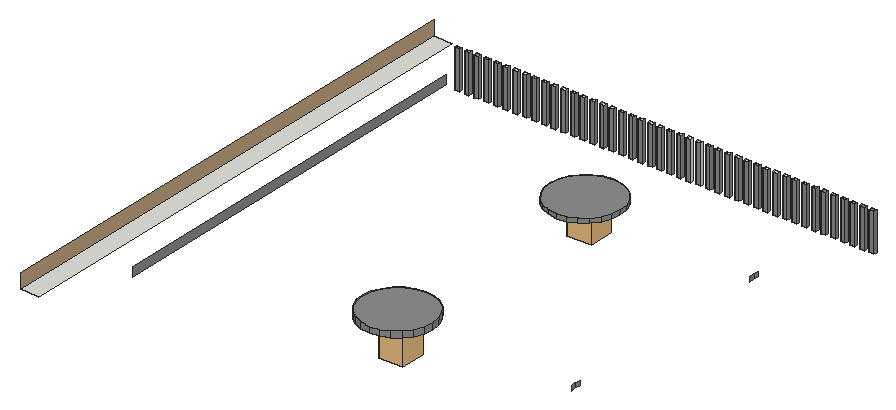
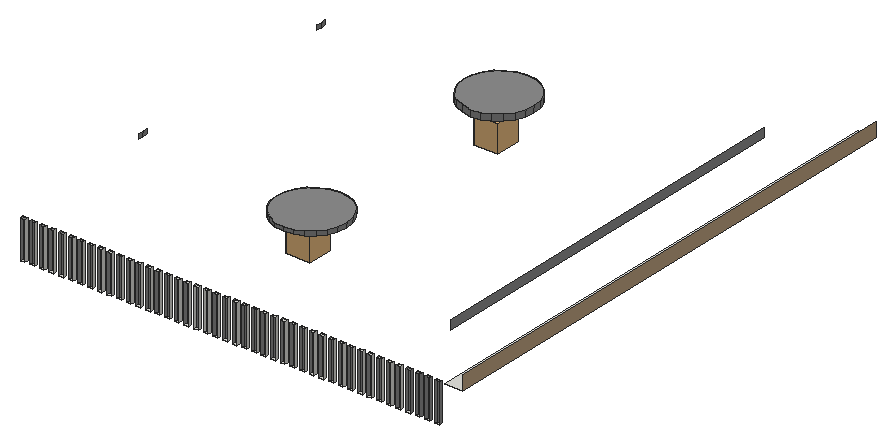
# SketchUp Ruby script. Lengths in inches.
U = 1.inch
M = Sketchup.active_model
def pt(a) = Geom::Point3d.new(a.map { |v| v * U })
def face(e, loops, mat)
  f = e.add_face(loops[0].map { |a| pt(a) })
  loops[1..].each { |l| e.add_face(l.map { |a| pt(a) }).erase! }
  f.material = f.back_material = mat if mat
  f
end
# faces: each face lists its corners as indices into pts; further lists are holes
def faces(e, pts, list, mat = nil) = list.each { |f| face(e, (f[0].is_a?(Array) ? f : [f]).map { |l| l.map { |i| pts[i] } }, mat) }
# xy, xz, yz: faces in a plane at the given z, y or x. An outline is a flat list of corners, or four numbers for a rectangle; further outlines are holes
def ring(l) = l.size == 4 ? [[l[0], l[1]], [l[2], l[1]], [l[2], l[3]], [l[0], l[3]]] : l.each_slice(2).to_a
def flat(e, list, mat, &to3) = list.each { |f| face(e, (f[0].is_a?(Array) ? f : [f]).map { |l| ring(l).map { |u, v| to3.(u, v) } }, mat) }
def xy(e, z, list, mat = nil) = flat(e, list, mat) { |x, y| [x, y, z] }
def xz(e, y, list, mat = nil) = flat(e, list, mat) { |x, z| [x, y, z] }
def yz(e, x, list, mat = nil) = flat(e, list, mat) { |y, z| [x, y, z] }
def lines(e, pts, list) = list.each { |a, b| e.add_line(pt(pts[a]), pt(pts[b])) }
# prism: a flat outline (further loops are holes) pulled along v
def prism(e, loops, v, mat = nil)
  f = face(e, loops, mat); d = Geom::Vector3d.new(v.map { |x| x * U })
  f.pushpull(f.normal.samedirection?(d) ? d.length : -d.length)
end
def box(e, o, s, mat = nil) = prism(e, [[o, [o[0] + s[0], o[1], o[2]], [o[0] + s[0], o[1] + s[1], o[2]], [o[0], o[1] + s[1], o[2]]]], [0, 0, s[2]], mat)
def at(x, y, z, deg = 0) = Geom::Transformation.translation(pt([x, y, z])) * Geom::Transformation.rotation(ORIGIN, Z_AXIS, deg.degrees)
def axes(o, x, y, z) = Geom::Transformation.new([*x, 0, *y, 0, *z, 0, *pt(o).to_a, 1])
def part(name) = M.definitions.add(name)
# library, detail: a bought-in or finely detailed component or shape, given as its bounding box
def library(name, o, s) = part(name).tap { |d| box(d.entities, o, s) }
def detail(e, o, s) = box(e.add_group.entities, o, s)
def put(e, d, t, mat = nil) = e.add_instance(d, t).tap { |i| i.material = mat if mat }
def group(e, t, mat = nil) = e.add_group.tap { |g| g.transformation = t; g.material = mat if mat }.entities
root = M.entities
M.materials.add("Sand A01 200cm").color = [193, 166, 131]
M.materials.add("[Color M04]").color = [142, 142, 142]
c1 = library("Spot Light\#4",[-5.1,-5.1,-11.05],[10.2,10.2,11.05])
c2 = library("Spot Light\#3",[-5.1,-5.1,-11.05],[10.2,10.2,11.05])
xy(root,222.8125,[[20.94,222.56,22.88,223.75],[24.91,222.56,26.85,223.75],[28.88,222.56,30.82,223.75],[32.85,222.56,34.79,223.75],[36.82,222.56,38.76,223.75],
  [40.79,222.56,42.73,223.75],[44.76,222.56,46.7,223.75],[48.73,222.56,50.67,223.75],[52.7,222.56,54.64,223.75],[56.67,222.56,58.61,223.75],
  [60.64,222.56,62.58,223.75],[64.6,222.56,66.55,223.75],[68.57,222.56,70.52,223.75],[72.54,222.56,74.49,223.75],[76.51,222.56,78.45,223.75],
  [80.48,222.56,82.42,223.75],[84.45,222.56,86.39,223.75],[88.42,222.56,90.36,223.75],[92.39,222.56,94.33,223.75],[96.36,222.56,98.3,223.75],
  [100.33,222.56,102.27,223.75],[104.3,222.56,106.24,223.75],[108.27,222.56,110.21,223.75],[112.24,222.56,114.18,223.75],[116.21,222.56,118.15,223.75],
  [120.18,222.56,122.12,223.75],[124.14,222.56,126.09,223.75],[128.11,222.56,130.06,223.75],[132.08,222.56,134.03,223.75],[136.05,222.56,137.99,223.75],
  [140.02,222.56,141.96,223.75],[143.99,222.56,145.93,223.75],[147.96,222.56,149.9,223.75],[151.93,222.56,153.87,223.75],[155.9,222.56,157.84,223.75],
  [159.87,222.56,161.81,223.75],[163.84,222.56,165.78,223.75],[167.81,222.56,169.75,223.75],[171.78,222.56,173.72,223.75],[175.75,222.56,177.6875,223.75],
  [179.71,222.56,181.66,223.75],[183.68,222.56,185.625,223.75],[187.65,222.56,189.6,223.75],[191.62,222.56,193.56,223.75]])
xy(root,238.625,[[11.13,11.13,18.94,223.75],[36.82,222.56,38.76,223.75],[40.79,222.56,42.73,223.75],[44.76,222.56,46.7,223.75],[48.73,222.56,50.67,223.75],
  [52.7,222.56,54.64,223.75],[56.67,222.56,58.61,223.75],[60.64,222.56,62.58,223.75],[64.6,222.56,66.55,223.75],[68.57,222.56,70.52,223.75],
  [72.54,222.56,74.49,223.75],[76.51,222.56,78.45,223.75],[80.48,222.56,82.42,223.75],[84.45,222.56,86.39,223.75],[88.42,222.56,90.36,223.75],
  [92.39,222.56,94.33,223.75],[96.36,222.56,98.3,223.75],[100.33,222.56,102.27,223.75],[104.3,222.56,106.24,223.75],[108.27,222.56,110.21,223.75],
  [112.24,222.56,114.18,223.75],[116.21,222.56,118.15,223.75],[120.18,222.56,122.12,223.75],[124.14,222.56,126.09,223.75],[128.11,222.56,130.06,223.75],
  [132.08,222.56,134.03,223.75],[136.05,222.56,137.99,223.75],[140.02,222.56,141.96,223.75],[143.99,222.56,145.93,223.75],[147.96,222.56,149.9,223.75],
  [151.93,222.56,153.87,223.75],[155.9,222.56,157.84,223.75],[159.87,222.56,161.81,223.75],[163.84,222.56,165.78,223.75]])
xy(root,238.625,[[20.94,222.56,22.88,223.75],[24.91,222.56,26.85,223.75],[28.88,222.56,30.82,223.75],[32.85,222.56,34.79,223.75],[167.81,222.56,169.75,223.75],
  [171.78,222.56,173.72,223.75],[175.75,222.56,177.6875,223.75],[179.71,222.56,181.66,223.75],[183.68,222.56,185.625,223.75],[187.65,222.56,189.6,223.75],
  [191.62,222.56,193.56,223.75]],"[Color M04]")
xy(root,242.625,[[119.36,152.06,115.61,152.55,112.11,154,109.11,156.31,106.8,159.31,105.35,162.81,104.86,166.56,105.35,170.3125,106.8,173.81,109.11,176.8125,112.11,179.12,115.61,180.57,119.36,181.06,123.11,180.57,126.61,179.12,129.61,176.8125,131.92,173.81,133.37,170.3125,133.86,166.56,133.37,162.81,131.92,159.31,129.61,156.31,126.61,154,123.11,152.55]],"[Color M04]")
xy(root,243.4375,[[119.36,55.56,115.61,56.05,112.11,57.5,109.11,59.81,106.8,62.81,105.35,66.31,104.86,70.06,105.35,73.8125,106.8,77.31,109.11,80.3125,112.11,82.62,115.61,84.07,119.36,84.56,123.11,84.07,126.61,82.62,129.61,80.3125,131.92,77.31,133.37,73.8125,133.86,70.06,133.37,66.31,131.92,62.81,129.61,59.81,126.61,57.5,123.11,56.05]],"[Color M04]")
xz(root,222.56,[[20.94,222.8125,22.88,238.625],[24.91,222.8125,26.85,238.625],[28.88,222.8125,30.82,238.625],[32.85,222.8125,34.79,238.625],[36.82,222.8125,38.76,238.625],
  [40.79,222.8125,42.73,238.625],[44.76,222.8125,46.7,238.625],[48.73,222.8125,50.67,238.625],[52.7,222.8125,54.64,238.625],[56.67,222.8125,58.61,238.625],
  [60.64,222.8125,62.58,238.625],[64.6,222.8125,66.55,238.625],[68.57,222.8125,70.52,238.625],[72.54,222.8125,74.49,238.625],[76.51,222.8125,78.45,238.625],
  [80.48,222.8125,82.42,238.625],[84.45,222.8125,86.39,238.625],[88.42,222.8125,90.36,238.625],[92.39,222.8125,94.33,238.625],[96.36,222.8125,98.3,238.625],
  [100.33,222.8125,102.27,238.625],[104.3,222.8125,106.24,238.625],[108.27,222.8125,110.21,238.625],[112.24,222.8125,114.18,238.625],[116.21,222.8125,118.15,238.625],
  [120.18,222.8125,122.12,238.625],[124.14,222.8125,126.09,238.625],[128.11,222.8125,130.06,238.625],[132.08,222.8125,134.03,238.625],[136.05,222.8125,137.99,238.625],
  [140.02,222.8125,141.96,238.625],[143.99,222.8125,145.93,238.625],[147.96,222.8125,149.9,238.625],[151.93,222.8125,153.87,238.625],[155.9,222.8125,157.84,238.625],
  [159.87,222.8125,161.81,238.625],[163.84,222.8125,165.78,238.625],[167.81,222.8125,169.75,238.625],[171.78,222.8125,173.72,238.625],[175.75,222.8125,177.6875,238.625],
  [179.71,222.8125,181.66,238.625],[183.68,222.8125,185.625,238.625],[187.65,222.8125,189.6,238.625],[191.62,222.8125,193.56,238.625]],"[Color M04]")
yz(root,11.13,[[11.13,238.625,223.75,244.625]],"Sand A01 200cm")
yz(root,20.94,[[222.56,222.8125,223.75,238.625]],"[Color M04]")
yz(root,22.88,[[222.56,222.8125,223.75,238.625]],"[Color M04]")
yz(root,24.91,[[222.56,222.8125,223.75,238.625]],"[Color M04]")
yz(root,26.85,[[222.56,222.8125,223.75,238.625]],"[Color M04]")
yz(root,28.88,[[222.56,222.8125,223.75,238.625]],"[Color M04]")
yz(root,30.82,[[222.56,222.8125,223.75,238.625]],"[Color M04]")
yz(root,32.85,[[222.56,222.8125,223.75,238.625]],"[Color M04]")
yz(root,34.79,[[222.56,222.8125,223.75,238.625]],"[Color M04]")
yz(root,36.82,[[222.56,222.8125,223.75,238.625]])
yz(root,36.86,[[36.86,240.875,198.01,244.625]],"[Color M04]")
yz(root,38.76,[[222.56,222.8125,223.75,238.625]],"[Color M04]")
yz(root,40.79,[[222.56,222.8125,223.75,238.625]])
yz(root,42.73,[[222.56,222.8125,223.75,238.625]],"[Color M04]")
yz(root,44.76,[[222.56,222.8125,223.75,238.625]])
yz(root,46.7,[[222.56,222.8125,223.75,238.625]],"[Color M04]")
yz(root,48.73,[[222.56,222.8125,223.75,238.625]])
yz(root,50.67,[[222.56,222.8125,223.75,238.625]],"[Color M04]")
yz(root,52.7,[[222.56,222.8125,223.75,238.625]])
yz(root,54.64,[[222.56,222.8125,223.75,238.625]],"[Color M04]")
yz(root,56.67,[[222.56,222.8125,223.75,238.625]])
yz(root,58.61,[[222.56,222.8125,223.75,238.625]],"[Color M04]")
yz(root,60.64,[[222.56,222.8125,223.75,238.625]])
yz(root,62.58,[[222.56,222.8125,223.75,238.625]],"[Color M04]")
yz(root,64.6,[[222.56,222.8125,223.75,238.625]])
yz(root,66.55,[[222.56,222.8125,223.75,238.625]],"[Color M04]")
yz(root,68.57,[[222.56,222.8125,223.75,238.625]])
yz(root,70.52,[[222.56,222.8125,223.75,238.625]],"[Color M04]")
yz(root,72.54,[[222.56,222.8125,223.75,238.625]])
yz(root,74.49,[[222.56,222.8125,223.75,238.625]],"[Color M04]")
yz(root,76.51,[[222.56,222.8125,223.75,238.625]])
yz(root,78.45,[[222.56,222.8125,223.75,238.625]],"[Color M04]")
yz(root,80.48,[[222.56,222.8125,223.75,238.625]])
yz(root,82.42,[[222.56,222.8125,223.75,238.625]],"[Color M04]")
yz(root,84.45,[[222.56,222.8125,223.75,238.625]])
yz(root,86.39,[[222.56,222.8125,223.75,238.625]],"[Color M04]")
yz(root,88.42,[[222.56,222.8125,223.75,238.625]])
yz(root,90.36,[[222.56,222.8125,223.75,238.625]],"[Color M04]")
yz(root,92.39,[[222.56,222.8125,223.75,238.625]])
yz(root,94.33,[[222.56,222.8125,223.75,238.625]],"[Color M04]")
yz(root,96.36,[[222.56,222.8125,223.75,238.625]])
yz(root,98.3,[[222.56,222.8125,223.75,238.625]],"[Color M04]")
yz(root,100.33,[[222.56,222.8125,223.75,238.625]])
yz(root,102.27,[[222.56,222.8125,223.75,238.625]],"[Color M04]")
yz(root,104.3,[[222.56,222.8125,223.75,238.625]])
yz(root,106.24,[[222.56,222.8125,223.75,238.625]],"[Color M04]")
yz(root,108.27,[[222.56,222.8125,223.75,238.625]])
yz(root,110.21,[[222.56,222.8125,223.75,238.625]],"[Color M04]")
yz(root,112.24,[[222.56,222.8125,223.75,238.625]])
yz(root,114.18,[[222.56,222.8125,223.75,238.625]],"[Color M04]")
yz(root,116.21,[[222.56,222.8125,223.75,238.625]])
yz(root,118.15,[[222.56,222.8125,223.75,238.625]])
yz(root,120.18,[[222.56,222.8125,223.75,238.625]])
yz(root,122.12,[[222.56,222.8125,223.75,238.625]])
yz(root,124.14,[[222.56,222.8125,223.75,238.625]])
yz(root,126.09,[[222.56,222.8125,223.75,238.625]],"[Color M04]")
yz(root,128.11,[[222.56,222.8125,223.75,238.625]])
yz(root,130.06,[[222.56,222.8125,223.75,238.625]],"[Color M04]")
yz(root,132.08,[[222.56,222.8125,223.75,238.625]])
yz(root,134.03,[[222.56,222.8125,223.75,238.625]],"[Color M04]")
yz(root,136.05,[[222.56,222.8125,223.75,238.625]])
yz(root,137.99,[[222.56,222.8125,223.75,238.625]],"[Color M04]")
yz(root,140.02,[[222.56,222.8125,223.75,238.625]])
yz(root,141.96,[[222.56,222.8125,223.75,238.625]],"[Color M04]")
yz(root,143.99,[[222.56,222.8125,223.75,238.625]])
yz(root,145.93,[[222.56,222.8125,223.75,238.625]],"[Color M04]")
yz(root,147.96,[[222.56,222.8125,223.75,238.625]])
yz(root,149.9,[[222.56,222.8125,223.75,238.625]],"[Color M04]")
yz(root,151.93,[[222.56,222.8125,223.75,238.625]])
yz(root,153.87,[[222.56,222.8125,223.75,238.625]],"[Color M04]")
yz(root,155.9,[[222.56,222.8125,223.75,238.625]])
yz(root,157.84,[[222.56,222.8125,223.75,238.625]],"[Color M04]")
yz(root,159.87,[[222.56,222.8125,223.75,238.625]])
yz(root,161.81,[[222.56,222.8125,223.75,238.625]],"[Color M04]")
yz(root,163.84,[[222.56,222.8125,223.75,238.625]])
yz(root,165.78,[[222.56,222.8125,223.75,238.625]],"[Color M04]")
yz(root,167.81,[[222.56,222.8125,223.75,238.625]])
yz(root,169.75,[[222.56,222.8125,223.75,238.625]],"[Color M04]")
yz(root,171.78,[[222.56,222.8125,223.75,238.625]])
yz(root,173.72,[[222.56,222.8125,223.75,238.625]],"[Color M04]")
yz(root,175.75,[[222.56,222.8125,223.75,238.625]])
yz(root,177.6875,[[222.56,222.8125,223.75,238.625]],"[Color M04]")
yz(root,179.71,[[222.56,222.8125,223.75,238.625]])
yz(root,181.66,[[222.56,222.8125,223.75,238.625]],"[Color M04]")
yz(root,183.68,[[222.56,222.8125,223.75,238.625]])
yz(root,185.625,[[222.56,222.8125,223.75,238.625]],"[Color M04]")
yz(root,187.65,[[222.56,222.8125,223.75,238.625]])
yz(root,189.6,[[222.56,222.8125,223.75,238.625]],"[Color M04]")
yz(root,191.62,[[222.56,222.8125,223.75,238.625]])
yz(root,193.56,[[222.56,222.8125,223.75,238.625]],"[Color M04]")
p = [[119.36,55.56,240.875],[115.61,56.05,240.875],[115.61,56.05,243.4375],[119.36,55.56,243.4375],[123.11,56.05,240.875],[123.11,56.05,243.4375],
  [112.11,57.5,240.875],[112.11,57.5,243.4375],[126.61,57.5,240.875],[126.61,57.5,243.4375],[109.11,59.81,240.875],[109.11,59.81,243.4375],
  [129.61,59.81,240.875],[129.61,59.81,243.4375],[106.8,62.81,240.875],[106.8,62.81,243.4375],[131.92,62.81,240.875],[131.92,62.81,243.4375],
  [105.35,66.31,240.875],[105.35,66.31,243.4375],[133.37,66.31,240.875],[133.37,66.31,243.4375],[104.86,70.06,240.875],[104.86,70.06,243.4375],
  [133.86,70.06,240.875],[133.86,70.06,243.4375],[193.71,66.81,240.875],[193.42,68.96,240.875],[193.42,68.96,242.5625],[193.71,66.81,242.5625],
  [193.71,71.11,240.875],[193.71,71.11,242.5625],[105.35,73.8125,240.875],[105.35,73.8125,243.4375],[133.37,73.8125,240.875],[133.37,73.8125,243.4375],
  [106.8,77.31,240.875],[106.8,77.31,243.4375],[131.92,77.31,240.875],[131.92,77.31,243.4375],[109.11,80.3125,240.875],[109.11,80.3125,243.4375],
  [129.61,80.3125,240.875],[129.61,80.3125,243.4375],[112.11,82.62,240.875],[112.11,82.62,243.4375],[126.61,82.62,240.875],[126.61,82.62,243.4375],
  [115.61,84.07,240.875],[115.61,84.07,243.4375],[123.11,84.07,240.875],[123.11,84.07,243.4375],[119.36,84.56,240.875],[119.36,84.56,243.4375],
  [119.36,152.06,240.875],[115.61,152.55,240.875],[115.61,152.55,242.625],[119.36,152.06,242.625],[123.11,152.55,240.875],[123.11,152.55,242.625],
  [112.11,154,240.875],[112.11,154,242.625],[126.61,154,240.875],[126.61,154,242.625],[109.11,156.31,240.875],[109.11,156.31,242.625],
  [129.61,156.31,240.875],[129.61,156.31,242.625],[106.8,159.31,240.875],[106.8,159.31,242.625],[131.92,159.31,240.875],[131.92,159.31,242.625],
  [193.71,158.5,240.875],[193.42,160.65,240.875],[193.42,160.65,242.75],[193.71,158.5,242.75],[105.35,162.81,240.875],[105.35,162.81,242.625],
  [133.37,162.81,240.875],[133.37,162.81,242.625],[193.71,162.8,240.875],[193.71,162.8,242.75],[104.86,166.56,240.875],[104.86,166.56,242.625],
  [133.86,166.56,240.875],[133.86,166.56,242.625],[105.35,170.3125,240.875],[105.35,170.3125,242.625],[133.37,170.3125,240.875],[133.37,170.3125,242.625],
  [106.8,173.81,240.875],[106.8,173.81,242.625],[131.92,173.81,240.875],[131.92,173.81,242.625],[109.11,176.8125,240.875],[109.11,176.8125,242.625],
  [129.61,176.8125,240.875],[129.61,176.8125,242.625],[112.11,179.12,240.875],[112.11,179.12,242.625],[126.61,179.12,240.875],[126.61,179.12,242.625],
  [115.61,180.57,240.875],[115.61,180.57,242.625],[123.11,180.57,240.875],[123.11,180.57,242.625],[119.36,181.06,240.875],[119.36,181.06,242.625]]
faces(root,p,[[0,1,2,3],[4,0,3,5],[1,6,7,2],[8,4,5,9],[6,10,11,7],[12,8,9,13],[10,14,15,11],[16,12,13,17],
  [14,18,19,15],[20,16,17,21],[18,22,23,19],[24,20,21,25],[26,27,28,29],[27,30,31,28],[22,32,33,23],[34,24,25,35],
  [32,36,37,33],[38,34,35,39],[36,40,41,37],[42,38,39,43],[40,44,45,41],[46,42,43,47],[44,48,49,45],[50,46,47,51],
  [48,52,53,49],[52,50,51,53],[54,55,56,57],[58,54,57,59],[55,60,61,56],[62,58,59,63],[60,64,65,61],[66,62,63,67],
  [64,68,69,65],[70,66,67,71],[72,73,74,75],[68,76,77,69],[78,70,71,79],[73,80,81,74],[76,82,83,77],[84,78,79,85],
  [82,86,87,83],[88,84,85,89],[86,90,91,87],[92,88,89,93],[90,94,95,91],[96,92,93,97],[94,98,99,95],[100,96,97,101],
  [98,102,103,99],[104,100,101,105],[102,106,107,103],[106,104,105,107]],"[Color M04]")
put(root,c1,at(119.36,168.52,238.86))
put(root,c2,at(119.36,71.71,236.37))
